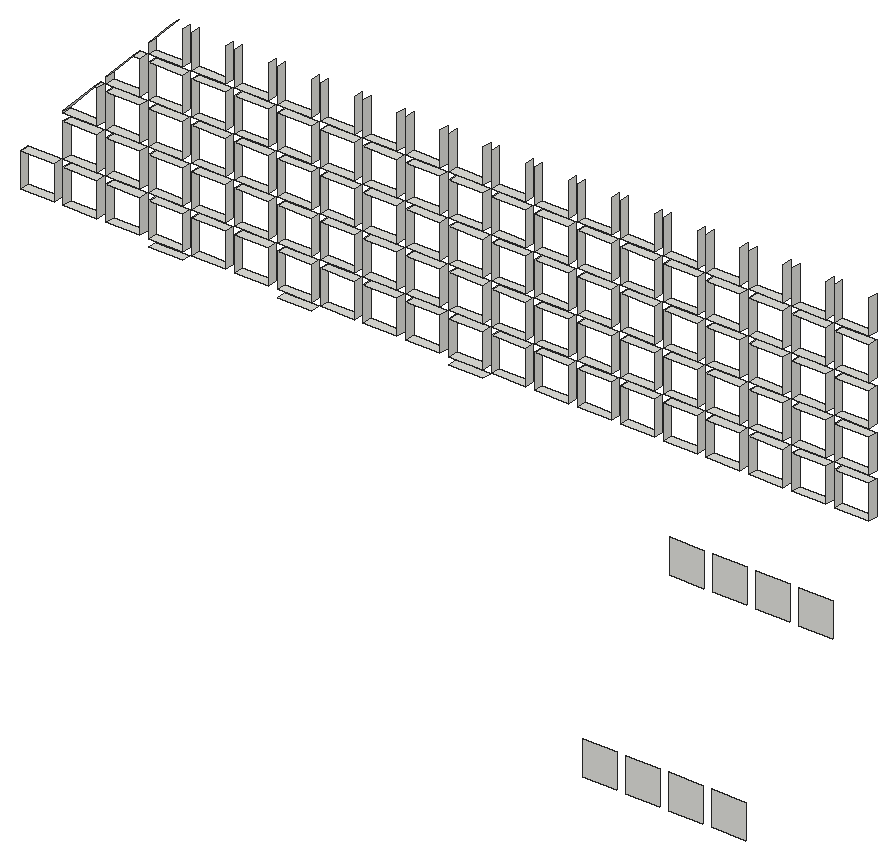
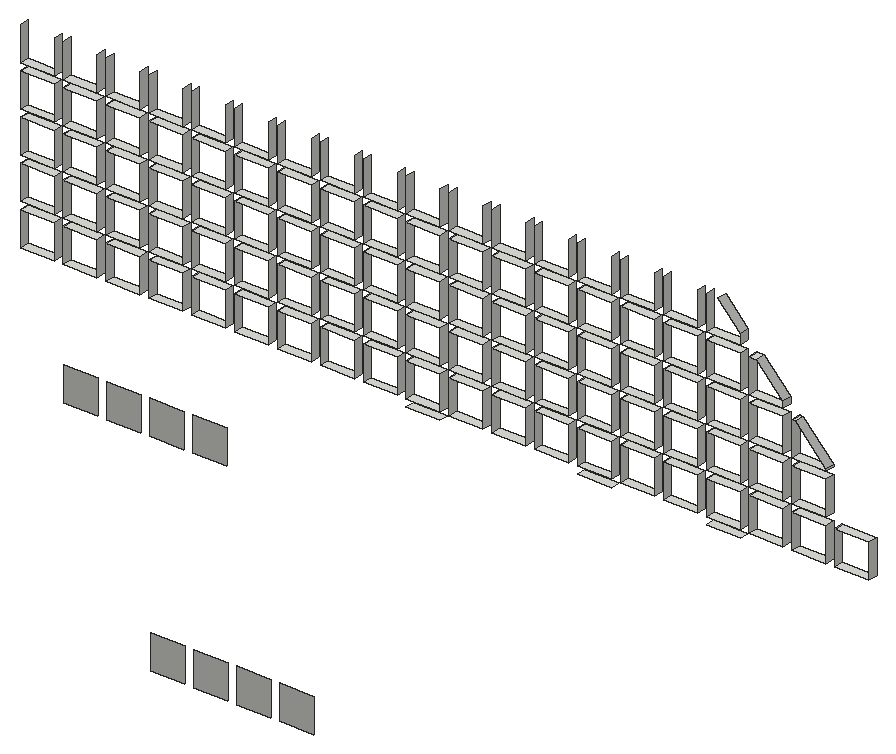
# SketchUp Ruby script. Lengths in inches.
U = 1.inch
M = Sketchup.active_model
def pt(a) = Geom::Point3d.new(a.map { |v| v * U })
def face(e, loops, mat)
  f = e.add_face(loops[0].map { |a| pt(a) })
  loops[1..].each { |l| e.add_face(l.map { |a| pt(a) }).erase! }
  f.material = f.back_material = mat if mat
  f
end
# faces: each face lists its corners as indices into pts; further lists are holes
def faces(e, pts, list, mat = nil) = list.each { |f| face(e, (f[0].is_a?(Array) ? f : [f]).map { |l| l.map { |i| pts[i] } }, mat) }
# xy, xz, yz: faces in a plane at the given z, y or x. An outline is a flat list of corners, or four numbers for a rectangle; further outlines are holes
def ring(l) = l.size == 4 ? [[l[0], l[1]], [l[2], l[1]], [l[2], l[3]], [l[0], l[3]]] : l.each_slice(2).to_a
def flat(e, list, mat, &to3) = list.each { |f| face(e, (f[0].is_a?(Array) ? f : [f]).map { |l| ring(l).map { |u, v| to3.(u, v) } }, mat) }
def xy(e, z, list, mat = nil) = flat(e, list, mat) { |x, y| [x, y, z] }
def xz(e, y, list, mat = nil) = flat(e, list, mat) { |x, z| [x, y, z] }
def yz(e, x, list, mat = nil) = flat(e, list, mat) { |y, z| [x, y, z] }
def lines(e, pts, list) = list.each { |a, b| e.add_line(pt(pts[a]), pt(pts[b])) }
# prism: a flat outline (further loops are holes) pulled along v
def prism(e, loops, v, mat = nil)
  f = face(e, loops, mat); d = Geom::Vector3d.new(v.map { |x| x * U })
  f.pushpull(f.normal.samedirection?(d) ? d.length : -d.length)
end
def box(e, o, s, mat = nil) = prism(e, [[o, [o[0] + s[0], o[1], o[2]], [o[0] + s[0], o[1] + s[1], o[2]], [o[0], o[1] + s[1], o[2]]]], [0, 0, s[2]], mat)
def at(x, y, z, deg = 0) = Geom::Transformation.translation(pt([x, y, z])) * Geom::Transformation.rotation(ORIGIN, Z_AXIS, deg.degrees)
def axes(o, x, y, z) = Geom::Transformation.new([*x, 0, *y, 0, *z, 0, *pt(o).to_a, 1])
def part(name) = M.definitions.add(name)
# library, detail: a bought-in or finely detailed component or shape, given as its bounding box
def library(name, o, s) = part(name).tap { |d| box(d.entities, o, s) }
def detail(e, o, s) = box(e.add_group.entities, o, s)
def put(e, d, t, mat = nil) = e.add_instance(d, t).tap { |i| i.material = mat if mat }
def group(e, t, mat = nil) = e.add_group.tap { |g| g.transformation = t; g.material = mat if mat }.entities
root = M.entities
xy(root,327.59,[[969.4,2332.13,971.71,2332.76],[978.14,2332.13,980.45,2332.76],[989.79,2332.13,992.1,2332.76]])
xy(root,328.09,[[960.67,2332.13,962.98,2332.76],[963.58,2332.13,965.89,2332.76],[966.49,2332.13,968.8,2332.76],[969.4,2332.13,971.71,2332.76],[972.3125,2332.13,974.625,2332.76],
  [975.23,2332.13,977.54,2332.76],[978.14,2332.13,980.45,2332.76],[981.05,2332.13,983.36,2332.76],[983.96,2332.13,986.27,2332.76],[986.875,2332.13,989.1875,2332.76],
  [989.79,2332.13,992.1,2332.76],[992.7,2332.13,995.01,2332.76],[995.61,2332.13,997.92,2332.76],[998.52,2332.13,1000.83,2332.76],[1001.43,2332.13,1003.75,2332.76],
  [1004.35,2332.13,1006.66,2332.76],[1007.26,2332.13,1009.57,2332.76],[1010.17,2332.13,1012.48,2332.76],[1013.08,2332.13,1015.4,2332.76],[1015.99,2332.13,1018.31,2332.76]])
xy(root,330.4,[[960.67,2332.13,962.98,2332.76],[963.58,2332.13,965.89,2332.76],[966.49,2332.13,968.8,2332.76],[969.4,2332.13,971.71,2332.76],[972.3125,2332.13,974.625,2332.76],
  [975.23,2332.13,977.54,2332.76],[978.14,2332.13,980.45,2332.76],[981.05,2332.13,983.36,2332.76],[983.96,2332.13,986.27,2332.76],[986.875,2332.13,989.1875,2332.76],
  [989.79,2332.13,992.1,2332.76],[992.7,2332.13,995.01,2332.76],[995.61,2332.13,997.92,2332.76],[998.52,2332.13,1000.83,2332.76],[1001.43,2332.13,1003.75,2332.76],
  [1004.35,2332.13,1006.66,2332.76],[1007.26,2332.13,1009.57,2332.76],[1010.17,2332.13,1012.48,2332.76],[1013.08,2332.13,1015.4,2332.76],[1015.99,2332.13,1018.31,2332.76]])
xy(root,330.9,[[963.58,2332.13,965.89,2332.76],[966.49,2332.13,968.8,2332.76],[969.4,2332.13,971.71,2332.76],[972.3125,2332.13,974.625,2332.76],[975.23,2332.13,977.54,2332.76],
  [978.14,2332.13,980.45,2332.76],[981.05,2332.13,983.36,2332.76],[983.96,2332.13,986.27,2332.76],[986.875,2332.13,989.1875,2332.76],[989.79,2332.13,992.1,2332.76],
  [992.7,2332.13,995.01,2332.76],[995.61,2332.13,997.92,2332.76],[998.52,2332.13,1000.83,2332.76],[1001.43,2332.13,1003.75,2332.76],[1004.35,2332.13,1006.66,2332.76],
  [1007.26,2332.13,1009.57,2332.76],[1010.17,2332.13,1012.48,2332.76],[1013.08,2332.13,1015.4,2332.76],[1015.99,2332.13,1018.31,2332.76]])
xy(root,333.21,[[963.58,2332.13,965.89,2332.76],[966.49,2332.13,968.8,2332.76],[969.4,2332.13,971.71,2332.76],[972.3125,2332.13,974.625,2332.76],[975.23,2332.13,977.54,2332.76],
  [978.14,2332.13,980.45,2332.76],[981.05,2332.13,983.36,2332.76],[983.96,2332.13,986.27,2332.76],[986.875,2332.13,989.1875,2332.76],[989.79,2332.13,992.1,2332.76],
  [992.7,2332.13,995.01,2332.76],[995.61,2332.13,997.92,2332.76],[998.52,2332.13,1000.83,2332.76],[1001.43,2332.13,1003.75,2332.76],[1004.35,2332.13,1006.66,2332.76],
  [1007.26,2332.13,1009.57,2332.76],[1010.17,2332.13,1012.48,2332.76],[1013.08,2332.13,1015.4,2332.76],[1015.99,2332.13,1018.31,2332.76]])
xy(root,333.71,[[963.58,2332.13,965.89,2332.76],[966.49,2332.13,968.8,2332.76],[969.4,2332.13,971.71,2332.76],[972.3125,2332.13,974.625,2332.76],[975.23,2332.13,977.54,2332.76],
  [978.14,2332.13,980.45,2332.76],[981.05,2332.13,983.36,2332.76],[983.96,2332.13,986.27,2332.76],[986.875,2332.13,989.1875,2332.76],[989.79,2332.13,992.1,2332.76],
  [992.7,2332.13,995.01,2332.76],[995.61,2332.13,997.92,2332.76],[998.52,2332.13,1000.83,2332.76],[1001.43,2332.13,1003.75,2332.76],[1004.35,2332.13,1006.66,2332.76],
  [1007.26,2332.13,1009.57,2332.76],[1010.17,2332.13,1012.48,2332.76],[1013.08,2332.13,1015.4,2332.76],[1015.99,2332.13,1018.31,2332.76]])
xy(root,336.02,[[965.64,2332.13,965.89,2332.76],[966.49,2332.13,968.8,2332.76],[969.4,2332.13,971.71,2332.76],[972.3125,2332.13,974.625,2332.76],[975.23,2332.13,977.54,2332.76],
  [978.14,2332.13,980.45,2332.76],[981.05,2332.13,983.36,2332.76],[983.96,2332.13,986.27,2332.76],[986.875,2332.13,989.1875,2332.76],[989.79,2332.13,992.1,2332.76],
  [992.7,2332.13,995.01,2332.76],[995.61,2332.13,997.92,2332.76],[998.52,2332.13,1000.83,2332.76],[1001.43,2332.13,1003.75,2332.76],[1004.35,2332.13,1006.66,2332.76],
  [1007.26,2332.13,1009.57,2332.76],[1010.17,2332.13,1012.48,2332.76],[1013.08,2332.13,1015.4,2332.76],[1015.99,2332.13,1018.31,2332.76]])
xy(root,336.52,[[966.49,2332.13,968.8,2332.76],[969.4,2332.13,971.71,2332.76],[972.3125,2332.13,974.625,2332.76],[975.23,2332.13,977.54,2332.76],[978.14,2332.13,980.45,2332.76],
  [981.05,2332.13,983.36,2332.76],[983.96,2332.13,986.27,2332.76],[986.875,2332.13,989.1875,2332.76],[989.79,2332.13,992.1,2332.76],[992.7,2332.13,995.01,2332.76],
  [995.61,2332.13,997.92,2332.76],[998.52,2332.13,1000.83,2332.76],[1001.43,2332.13,1003.75,2332.76],[1004.35,2332.13,1006.66,2332.76],[1007.26,2332.13,1009.57,2332.76],
  [1010.17,2332.13,1012.48,2332.76],[1013.08,2332.13,1015.4,2332.76],[1015.99,2332.13,1018.31,2332.76]])
xy(root,338.84,[[968.28,2332.13,968.8,2332.76],[969.4,2332.13,971.71,2332.76],[972.3125,2332.13,974.625,2332.76],[975.23,2332.13,977.54,2332.76],[978.14,2332.13,980.45,2332.76],
  [981.05,2332.13,983.36,2332.76],[983.96,2332.13,986.27,2332.76],[986.875,2332.13,989.1875,2332.76],[989.79,2332.13,992.1,2332.76],[992.7,2332.13,995.01,2332.76],
  [995.61,2332.13,997.92,2332.76],[998.52,2332.13,1000.83,2332.76],[1001.43,2332.13,1003.75,2332.76],[1004.35,2332.13,1006.66,2332.76],[1007.26,2332.13,1009.57,2332.76],
  [1010.17,2332.13,1012.48,2332.76],[1013.08,2332.13,1015.4,2332.76],[1015.99,2332.13,1018.31,2332.76]])
xy(root,339.34,[[969.4,2332.13,971.71,2332.76],[972.3125,2332.13,974.625,2332.76],[975.23,2332.13,977.54,2332.76],[978.14,2332.13,980.45,2332.76],[981.05,2332.13,983.36,2332.76],
  [983.96,2332.13,986.27,2332.76],[986.875,2332.13,989.1875,2332.76],[989.79,2332.13,992.1,2332.76],[992.7,2332.13,995.01,2332.76],[995.61,2332.13,997.92,2332.76],
  [998.52,2332.13,1000.83,2332.76],[1001.43,2332.13,1003.75,2332.76],[1004.35,2332.13,1006.66,2332.76],[1007.26,2332.13,1009.57,2332.76],[1010.17,2332.13,1012.48,2332.76],
  [1013.08,2332.13,1015.4,2332.76],[1015.99,2332.13,1018.31,2332.76]])
xz(root,2332.63,[[998.49,305.35,1000.81,307.67],[1001.41,305.35,1003.72,307.67],[1004.32,305.35,1006.63,307.67],[1007.23,305.35,1009.54,307.67]])
xz(root,2332.7,[[1004.35,319.65,1006.66,321.96],[1007.26,319.65,1009.57,321.96],[1010.17,319.65,1012.48,321.96],[1013.08,319.65,1015.4,321.96]])
yz(root,960.67,[[2332.13,328.09,2332.76,330.4]])
yz(root,962.98,[[2332.13,328.09,2332.76,330.4]])
yz(root,963.58,[[2332.13,328.09,2332.76,330.4],[2332.13,330.9,2332.76,333.21],[2332.13,333.71,2332.76,333.82]])
yz(root,965.89,[[2332.13,328.09,2332.76,330.4],[2332.13,330.9,2332.76,333.21],[2332.13,333.71,2332.76,336.02]])
yz(root,966.49,[[2332.13,328.09,2332.76,330.4],[2332.13,330.9,2332.76,333.21],[2332.13,333.71,2332.76,336.02],[2332.13,336.52,2332.76,336.93]])
yz(root,968.8,[[2332.13,328.09,2332.76,330.4],[2332.13,330.9,2332.76,333.21],[2332.13,333.71,2332.76,336.02],[2332.13,336.52,2332.76,338.84]])
yz(root,969.4,[[2332.13,328.09,2332.76,330.4],[2332.13,330.9,2332.76,333.21],[2332.13,333.71,2332.76,336.02],[2332.13,336.52,2332.76,338.84],[2332.13,339.34,2332.76,340.04]])
yz(root,971.71,[[2332.13,328.09,2332.76,330.4],[2332.13,330.9,2332.76,333.21],[2332.13,333.71,2332.76,336.02],[2332.13,336.52,2332.76,338.84],[2332.13,339.34,2332.76,341.65]])
yz(root,972.3125,[[2332.13,328.09,2332.76,330.4],[2332.13,330.9,2332.76,333.21],[2332.13,333.71,2332.76,336.02],[2332.13,336.52,2332.76,338.84],[2332.13,339.34,2332.76,341.65]])
yz(root,974.625,[[2332.13,328.09,2332.76,330.4],[2332.13,330.9,2332.76,333.21],[2332.13,333.71,2332.76,336.02],[2332.13,336.52,2332.76,338.84],[2332.13,339.34,2332.76,341.65]])
yz(root,975.23,[[2332.13,328.09,2332.76,330.4],[2332.13,330.9,2332.76,333.21],[2332.13,333.71,2332.76,336.02],[2332.13,336.52,2332.76,338.84],[2332.13,339.34,2332.76,341.65]])
yz(root,977.54,[[2332.13,328.09,2332.76,330.4],[2332.13,330.9,2332.76,333.21],[2332.13,333.71,2332.76,336.02],[2332.13,336.52,2332.76,338.84],[2332.13,339.34,2332.76,341.65]])
yz(root,978.14,[[2332.13,328.09,2332.76,330.4],[2332.13,330.9,2332.76,333.21],[2332.13,333.71,2332.76,336.02],[2332.13,336.52,2332.76,338.84],[2332.13,339.34,2332.76,341.65]])
yz(root,980.45,[[2332.13,328.09,2332.76,330.4],[2332.13,330.9,2332.76,333.21],[2332.13,333.71,2332.76,336.02],[2332.13,336.52,2332.76,338.84],[2332.13,339.34,2332.76,341.65]])
yz(root,981.05,[[2332.13,328.09,2332.76,330.4],[2332.13,330.9,2332.76,333.21],[2332.13,333.71,2332.76,336.02],[2332.13,336.52,2332.76,338.84],[2332.13,339.34,2332.76,341.65]])
yz(root,983.36,[[2332.13,328.09,2332.76,330.4],[2332.13,330.9,2332.76,333.21],[2332.13,333.71,2332.76,336.02],[2332.13,336.52,2332.76,338.84],[2332.13,339.34,2332.76,341.65]])
yz(root,983.96,[[2332.13,328.09,2332.76,330.4],[2332.13,330.9,2332.76,333.21],[2332.13,333.71,2332.76,336.02],[2332.13,336.52,2332.76,338.84],[2332.13,339.34,2332.76,341.65]])
yz(root,986.27,[[2332.13,328.09,2332.76,330.4],[2332.13,330.9,2332.76,333.21],[2332.13,333.71,2332.76,336.02],[2332.13,336.52,2332.76,338.84],[2332.13,339.34,2332.76,341.65]])
yz(root,986.875,[[2332.13,328.09,2332.76,330.4],[2332.13,330.9,2332.76,333.21],[2332.13,333.71,2332.76,336.02],[2332.13,336.52,2332.76,338.84],[2332.13,339.34,2332.76,341.65]])
yz(root,989.1875,[[2332.13,328.09,2332.76,330.4],[2332.13,330.9,2332.76,333.21],[2332.13,333.71,2332.76,336.02],[2332.13,336.52,2332.76,338.84],[2332.13,339.34,2332.76,341.65]])
yz(root,989.79,[[2332.13,328.09,2332.76,330.4],[2332.13,330.9,2332.76,333.21],[2332.13,333.71,2332.76,336.02],[2332.13,336.52,2332.76,338.84],[2332.13,339.34,2332.76,341.65]])
yz(root,992.1,[[2332.13,328.09,2332.76,330.4],[2332.13,330.9,2332.76,333.21],[2332.13,333.71,2332.76,336.02],[2332.13,336.52,2332.76,338.84],[2332.13,339.34,2332.76,341.65]])
yz(root,992.7,[[2332.13,328.09,2332.76,330.4],[2332.13,330.9,2332.76,333.21],[2332.13,333.71,2332.76,336.02],[2332.13,336.52,2332.76,338.84],[2332.13,339.34,2332.76,341.65]])
yz(root,995.01,[[2332.13,328.09,2332.76,330.4],[2332.13,330.9,2332.76,333.21],[2332.13,333.71,2332.76,336.02],[2332.13,336.52,2332.76,338.84],[2332.13,339.34,2332.76,341.65]])
yz(root,995.61,[[2332.13,328.09,2332.76,330.4],[2332.13,330.9,2332.76,333.21],[2332.13,333.71,2332.76,336.02],[2332.13,336.52,2332.76,338.84],[2332.13,339.34,2332.76,341.65]])
yz(root,997.92,[[2332.13,328.09,2332.76,330.4],[2332.13,330.9,2332.76,333.21],[2332.13,333.71,2332.76,336.02],[2332.13,336.52,2332.76,338.84],[2332.13,339.34,2332.76,341.65]])
yz(root,998.52,[[2332.13,328.09,2332.76,330.4],[2332.13,330.9,2332.76,333.21],[2332.13,333.71,2332.76,336.02],[2332.13,336.52,2332.76,338.84],[2332.13,339.34,2332.76,341.65]])
yz(root,1000.83,[[2332.13,328.09,2332.76,330.4],[2332.13,330.9,2332.76,333.21],[2332.13,333.71,2332.76,336.02],[2332.13,336.52,2332.76,338.84],[2332.13,339.34,2332.76,341.65]])
yz(root,1001.43,[[2332.13,328.09,2332.76,330.4],[2332.13,330.9,2332.76,333.21],[2332.13,333.71,2332.76,336.02],[2332.13,336.52,2332.76,338.84],[2332.13,339.34,2332.76,341.65]])
yz(root,1003.75,[[2332.13,328.09,2332.76,330.4],[2332.13,330.9,2332.76,333.21],[2332.13,333.71,2332.76,336.02],[2332.13,336.52,2332.76,338.84],[2332.13,339.34,2332.76,341.65]])
yz(root,1004.35,[[2332.13,328.09,2332.76,330.4],[2332.13,330.9,2332.76,333.21],[2332.13,333.71,2332.76,336.02],[2332.13,336.52,2332.76,338.84],[2332.13,339.34,2332.76,341.65]])
yz(root,1006.66,[[2332.13,328.09,2332.76,330.4],[2332.13,330.9,2332.76,333.21],[2332.13,333.71,2332.76,336.02],[2332.13,336.52,2332.76,338.84],[2332.13,339.34,2332.76,341.65]])
yz(root,1007.26,[[2332.13,328.09,2332.76,330.4],[2332.13,330.9,2332.76,333.21],[2332.13,333.71,2332.76,336.02],[2332.13,336.52,2332.76,338.84],[2332.13,339.34,2332.76,341.65]])
yz(root,1009.57,[[2332.13,328.09,2332.76,330.4],[2332.13,330.9,2332.76,333.21],[2332.13,333.71,2332.76,336.02],[2332.13,336.52,2332.76,338.84],[2332.13,339.34,2332.76,341.65]])
yz(root,1010.17,[[2332.13,328.09,2332.76,330.4],[2332.13,330.9,2332.76,333.21],[2332.13,333.71,2332.76,336.02],[2332.13,336.52,2332.76,338.84],[2332.13,339.34,2332.76,341.65]])
yz(root,1012.48,[[2332.13,328.09,2332.76,330.4],[2332.13,330.9,2332.76,333.21],[2332.13,333.71,2332.76,336.02],[2332.13,336.52,2332.76,338.84],[2332.13,339.34,2332.76,341.65]])
yz(root,1013.08,[[2332.13,328.09,2332.76,330.4],[2332.13,330.9,2332.76,333.21],[2332.13,333.71,2332.76,336.02],[2332.13,336.52,2332.76,338.84],[2332.13,339.34,2332.76,341.65]])
yz(root,1015.4,[[2332.13,328.09,2332.76,330.4],[2332.13,330.9,2332.76,333.21],[2332.13,333.71,2332.76,336.02],[2332.13,336.52,2332.76,338.84],[2332.13,339.34,2332.76,341.65]])
yz(root,1015.99,[[2332.13,328.09,2332.76,330.4],[2332.13,330.9,2332.76,333.21],[2332.13,333.71,2332.76,336.02],[2332.13,336.52,2332.76,338.84],[2332.13,339.34,2332.76,341.65]])
yz(root,1018.31,[[2332.13,328.09,2332.76,330.4],[2332.13,330.9,2332.76,333.21],[2332.13,333.71,2332.76,336.02],[2332.13,336.52,2332.76,338.84],[2332.13,339.34,2332.76,341.65]])
p = [[965.64,2332.13,336.02],[963.58,2332.13,333.82],[963.58,2332.76,333.82],[965.64,2332.76,336.02],[968.28,2332.13,338.84],[966.49,2332.13,336.93],
  [966.49,2332.76,336.93],[968.28,2332.76,338.84],[970.91,2332.13,341.65],[969.4,2332.13,340.04],[969.4,2332.76,340.04],[970.91,2332.76,341.65]]
faces(root,p,[[0,1,2,3],[4,5,6,7],[8,9,10,11]])
